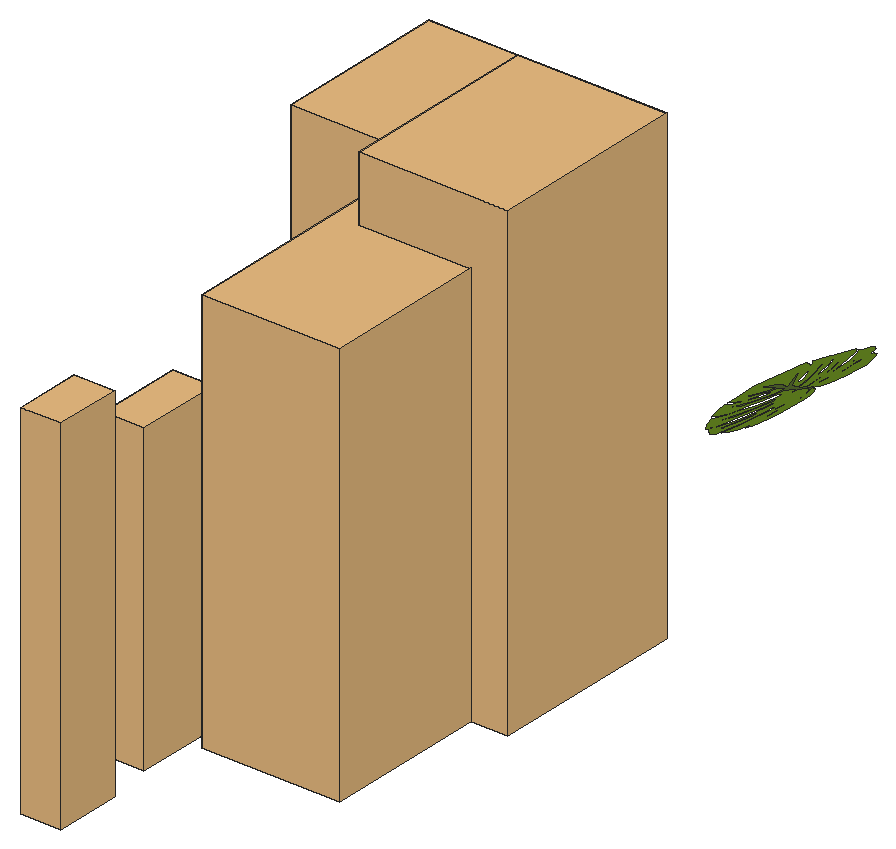
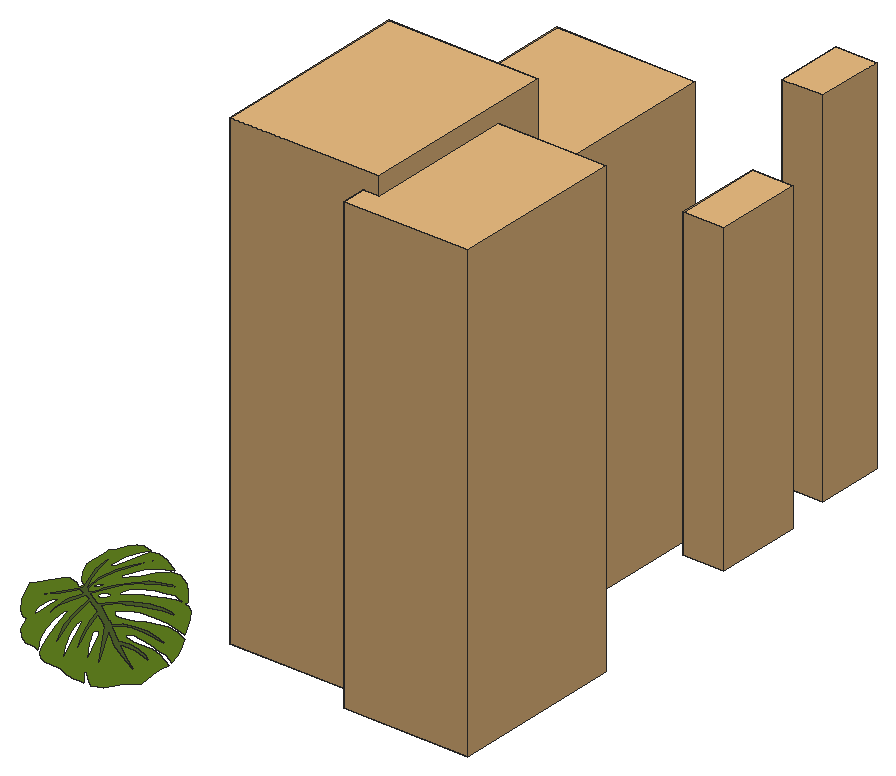
# SketchUp Ruby script. Lengths in inches.
U = 1.inch
M = Sketchup.active_model
def pt(a) = Geom::Point3d.new(a.map { |v| v * U })
def face(e, loops, mat)
  f = e.add_face(loops[0].map { |a| pt(a) })
  loops[1..].each { |l| e.add_face(l.map { |a| pt(a) }).erase! }
  f.material = f.back_material = mat if mat
  f
end
# faces: each face lists its corners as indices into pts; further lists are holes
def faces(e, pts, list, mat = nil) = list.each { |f| face(e, (f[0].is_a?(Array) ? f : [f]).map { |l| l.map { |i| pts[i] } }, mat) }
# xy, xz, yz: faces in a plane at the given z, y or x. An outline is a flat list of corners, or four numbers for a rectangle; further outlines are holes
def ring(l) = l.size == 4 ? [[l[0], l[1]], [l[2], l[1]], [l[2], l[3]], [l[0], l[3]]] : l.each_slice(2).to_a
def flat(e, list, mat, &to3) = list.each { |f| face(e, (f[0].is_a?(Array) ? f : [f]).map { |l| ring(l).map { |u, v| to3.(u, v) } }, mat) }
def xy(e, z, list, mat = nil) = flat(e, list, mat) { |x, y| [x, y, z] }
def xz(e, y, list, mat = nil) = flat(e, list, mat) { |x, z| [x, y, z] }
def yz(e, x, list, mat = nil) = flat(e, list, mat) { |y, z| [x, y, z] }
def lines(e, pts, list) = list.each { |a, b| e.add_line(pt(pts[a]), pt(pts[b])) }
# prism: a flat outline (further loops are holes) pulled along v
def prism(e, loops, v, mat = nil)
  f = face(e, loops, mat); d = Geom::Vector3d.new(v.map { |x| x * U })
  f.pushpull(f.normal.samedirection?(d) ? d.length : -d.length)
end
def box(e, o, s, mat = nil) = prism(e, [[o, [o[0] + s[0], o[1], o[2]], [o[0] + s[0], o[1] + s[1], o[2]], [o[0], o[1] + s[1], o[2]]]], [0, 0, s[2]], mat)
def at(x, y, z, deg = 0) = Geom::Transformation.translation(pt([x, y, z])) * Geom::Transformation.rotation(ORIGIN, Z_AXIS, deg.degrees)
def axes(o, x, y, z) = Geom::Transformation.new([*x, 0, *y, 0, *z, 0, *pt(o).to_a, 1])
def part(name) = M.definitions.add(name)
# library, detail: a bought-in or finely detailed component or shape, given as its bounding box
def library(name, o, s) = part(name).tap { |d| box(d.entities, o, s) }
def detail(e, o, s) = box(e.add_group.entities, o, s)
def put(e, d, t, mat = nil) = e.add_instance(d, t).tap { |i| i.material = mat if mat }
def group(e, t, mat = nil) = e.add_group.tap { |g| g.transformation = t; g.material = mat if mat }.entities
root = M.entities
M.materials.add("[0059_DarkOliveGreen]").color = [85, 107, 47]
M.materials.add("[0061_OliveDrab]").color = [107, 142, 35]
c1 = library("EXOTIC-PEONY",[-0.63,-0.48,-0.08],[13.23,10.24,55.71])
c2 = library("EXOTIC-RED-POKER\#1",[-1.18,-1.18,0],[10.24,10.24,66.04])
c3 = library("EXOTICA-CAT-TAIL",[-18.64,-20.64,0],[26.41,31.25,82.25])
c4 = library("EXOTIC-BAMBOO",[-8.14,-8.14,0],[38.48,34.74,73.65])
c5 = library("EXOTIC-BAMBOO-TOO",[-9.25,-15.15,0],[30.31,37.46,85.46])
p = [[300.68,91.1875,26.91],[300.57,90.58,26.85],[301.02,90.23,27.08],[301.65,89.36,27.4],[302.04,88.16,27.6],[302.1,86.89,27.63],
  [302.04,85.61,27.6],[302.09,84.71,27.62],[301.77,83.65,27.46],[301.54,82.48,27.34],[301.15,81.46,27.15],[300.68,80.95,26.91],
  [300,80.7,26.56],[300.21,81.47,26.67],[300.48,82.51,26.81],[300.7,83.8,26.92],[300.83,85.63,26.99],[300.82,85.94,26.98],
  [300.67,86.03,26.9],[300.54,85.72,26.84],[300.38,84.69,26.76],[300.26,83.26,26.7],[299.99,81.49,26.5625],[299.89,80.92,26.51],
  [299.39,80.3125,26.26],[298.5,80.1,25.81],[297.26,80.46,25.18],[298.28,82.12,25.7],[298.82,83.32,25.97],[299.28,85.14,26.2],
  [299.37,86.05,26.25],[299.28,86.26,26.2],[299.1,86.03,26.11],[298.92,85.41,26.02],[298.47,84.05,25.79],[298.03,82.48,25.57],
  [297.32,81.02,25.21],[296.71,80.39,24.9],[295.62,80.625,24.35],[294.96,81.31,24.02],[294.23,82.125,23.65],[294.08,82.44,23.57],
  [294.29,82.8,23.68],[294.79,82.82,23.93],[295.17,82.96,24.13],[295.84,83.54,24.46],[296.53,84.29,24.8125],[297.58,85.77,25.34],
  [297.97,86.72,25.54],[298.09,87.53,25.6],[298.07,87.98,25.59],[297.86,87.94,25.48],[297.69,87.54,25.4],[297.31,86.81,25.21],
  [296.81,85.875,24.96],[296.04,84.78,24.57],[295.51,84.06,24.3],[294.875,83.22,23.98],[293.66,82.7,23.36],[293.24,82.91,23.15],
  [292.625,83.96,22.84],[291.67,85.875,22.36],[293.25,86.39,23.16],[294.5,87.09,23.79],[295.52,87.9,24.3],[296.32,88.89,24.71],
  [296.67,89.64,24.88],[296.87,90.27,24.99],[296.65,90.59,24.875],[296.3125,90.54,24.7],[295.83,90.05,24.46],[295.25,89.29,24.17],
  [294.59,88.34,23.83],[293.625,87.25,23.35],[293.06,86.76,23.06],[292.27,86.41,22.66],[291.2,86.44,22.125],[290.97,87.03,22.01],
  [290.75,87.49,21.89],[290.5,88.1,21.77],[290.26,88.87,21.64],[290.08,89.94,21.56],[290.51,89.78,21.77],[290.98,89.73,22.01],
  [291.53,89.94,22.29],[292.45,90.18,22.75],[293.51,90.53,23.29],[293.96,90.82,23.51],[294.4,91.29,23.74],[294.49,91.55,23.78],
  [294.39,91.72,23.73],[294.05,91.67,23.5625],[293.64,91.61,23.35],[293.01,91.11,23.04],[292.09,90.47,22.57],[291.26,90.34,22.15],
  [289.97,90.52,21.5],[290.01,91.46,21.52],[290,93.02,21.52],[289.79,94.92,21.41],[290.81,97.07,21.93],[291.35,98.88,22.2],
  [291.74,99.41,22.4],[292.14,99.93,22.6],[292.38,99.9,22.72],[293.87,98.72,23.47],[293.22,99.68,23.14],[292.78,100.3,22.92],
  [293.08,100.48,23.07],[293.6,100.88,23.34],[294.22,101.11,23.65],[294.88,101.1,23.98],[295.17,101.27,24.125],[295.73,101.61,24.41],
  [296.37,101.93,24.73],[296.82,102.01,24.96],[297.3,101.58,25.2],[297.66,100.75,25.38],[298.22,99.01,25.67],[298.68,97.28,25.9],
  [299.08,95.14,26.1],[299.2,94.75,26.16],[299.29,94.77,26.21],[299.33,95.16,26.23],[299.25,96.75,26.1875],[298.89,98.52,26.01],
  [298.37,100.14,25.74],[297.67,101.4,25.39],[297.98,101.44,25.54],[298.78,101.78,25.95],[299.39,101.65,26.26],[300.15,100.89,26.64],
  [300.57,99.39,26.86],[301.02,99.46,27.08],[301.66,99.11,27.41],[302.41,97.9375,27.78],[303.37,95.52,28.27],[303.04,94.67,28.1],
  [302.65,93.35,27.91],[302.22,91.93,27.6875],[301.79,91.16,27.47],[301.16,91.0625,27.16],[296.2,92.67,24.65],[293.7,96.79,23.39],
  [295.625,92.74,24.36],[294.3,93.61,23.6875],[293,94.02,23.03],[291.58,94.19,22.3125],[291.45,94.2,22.25],[292.31,93.91,22.68],
  [292.95,93.63,23.01],[294.16,93.14,23.62],[293.58,92.64,23.32],[292.78,92.13,22.92],[291.44,91.92,22.24],[291.99,91.66,22.52],
  [292.79,91.78,22.93],[293.63,92.16,23.35],[294.41,92.86,23.74],[295.85,92.03,24.47],[295.375,91.02,24.23],[294.6875,90.16,23.88],
  [293.78,89.52,23.43],[292.03,88.72,22.54],[293.02,88.87,23.04],[293.81,89.19,23.4375],[294.74,89.82,23.91],[295.54,90.73,24.32],
  [296.01,91.8,24.55],[298,90.95,25.56],[297.37,89.26,25.24],[295.93,87.08,24.51],[294.66,85.62,23.87],[293.79,84.89,23.43],
  [294.18,84.95,23.63],[294.85,85.38,23.96],[295.77,86.15,24.43],[297.29,88.25,25.2],[297.84,89.57,25.47],[298.4,91.01,25.76],
  [299.53,90.73,26.33],[299.02,88.52,26.07],[298.48,86.625,25.8],[297.7,84.74,25.4],[297.13,83.68,25.12],[295.93,82.11,24.51],
  [296.31,82.17,24.71],[296.93,82.99,25.02],[297.71,83.97,25.41],[298.35,85.35,25.73],[299.17,87.77,26.15],[299.4,88.7,26.27],
  [299.49,89.66,26.31],[299.67,90.47,26.4],[299.83,90.62,26.48],[300.03,90.41,26.58],[300.125,89.72,26.63],[300.2,88.31,26.67],
  [299.97,86.1875,26.55],[299.68,84.41,26.41],[299.08,81.59,26.1],[299.375,82.35,26.25],[299.84,84.03,26.49],[300.21,85.81,26.67],
  [300.45,88.41,26.79],[300.19,90.34,26.67],[300.54,89.43,26.84],[301.01,87.58,27.08],[301.41,85.07,27.28],[301.4375,86.21,27.29],
  [301.28,87.85,27.21],[300.68,89.88,26.91],[300.45,90.92,26.79],[302.14,96.12,27.65],[301.09,93.83,27.12],[300.38,91.45,26.76],
  [299.97,91.39,26.55],[299.95,91.78,26.54],[300.36,93.36,26.75],[300.25,95.54,26.69],[299.82,97.98,26.47],[300.11,94.95,26.625],
  [299.8125,92.92,26.47],[299.59,91.38,26.36],[299.18,91.55,26.15],[298.87,93.96,25.99],[298.34,96.54,25.73],[297.07,99.64,25.09],
  [298.3,95.18,25.71],[298.9,91.71,26.01],[297.8125,91.98,25.46],[297.45,93.43,25.28],[296.59,95.91,24.84],[295.47,98.28,24.28],
  [296.77,94.7,24.93],[297.41,92.22,25.26],[297.33,96.77,25.22],[296.84,97.91,24.97],[296.5625,98.54,24.83],[295.44,100.46,24.27],
  [295.74,99.71,24.42],[296.39,98.13,24.74],[296.95,96.54,25.03],[297.45,95.1,25.28],[297.67,94.49,25.39],[297.79,94.42,25.45],
  [297.84,94.64,25.48],[297.8,95.16,25.45],[295.91,95.31,24.5],[295.75,95.64,24.42],[295.6,95.95,24.34],[294.43,97.8,23.75],
  [295.01,96.29,24.04],[295.63,94.66,24.36],[295.78,94.25,24.4375],[296.05,93.85,24.57],[296.24,93.78,24.67],[296.36,94.04,24.73],
  [296.23,94.67,24.66],[301.05,96.1,27.1],[301.0625,96.64,27.1],[300.93,97.5625,27.04],[300.63,98.09,26.88],[300.58,97.74,26.86],
  [300.5625,96.3,26.85],[300.61,94.57,26.875],[300.74,94.52,26.94],[300.92,94.76,27.03],[301.04,95.55,27.09],[298.79,90.34,25.95],
  [298.45,89.9,25.79],[298.35,89.26,25.73],[298.47,89,25.79],[298.76,89.16,25.94],[298.99,89.64,26.06],[299.04,90.24,26.08],
  [299.87,89.05,26.5],[299.98,89.49,26.56],[299.87,89.8125,26.5],[299.67,89.44,26.4],[299.5,88.77,26.3125],[299.625,88.53,26.38],
  [299.82,88.86,26.48]]
faces(root,p,[[[0,1,2,3,4,5,6,7,8,9,10,11,12,13,14,15,16,17,18,19,20,21,22,23,24,25,26,27,28,29,30,31,32,33,34,35,36,37,38,39,40,41,42,43,44,45,46,47,48,49,50,51,52,53,54,55,56,57,42,58,59,60,61,62,63,64,65,66,67,68,69,70,71,72,73,74,75,76,77,78,79,80,81,82,83,84,85,86,87,88,89,90,91,92,93,94,95,96,97,98,99,100,101,102,103,104,105,106,107,108,109,110,111,112,113,114,115,116,117,118,119,120,121,122,123,124,125,126,127,128,129,130,131,132,133,134,135,136,137,138,139,140,141],[142,143,144,145,146,147,148,149,150,151,152,153,154,155,156,157,158,159,160,161,162,163,164,165,166,167,168,169,170,171,172,173,174,175,176,177,178,179,180,181,182,183,184,185,186,187,188,189,190,191,192,193,194,195,196,197,198,199,200,201,202,203,204,205,206,207,208,209,210,211,212,213,214,215,216,217,218,219,220,221,222,223,224,225,226,227,228,229,230,231,232,233,234,235],[236,237,238,239,240,241,242,243,244,245,246,247],[248,249,250,251,252,253,254,255,256,257,258],[259,260,261,262,263,264,265,266,267,268],[269,270,271,272,273,274,275],[276,277,278,279,280,281,282]]],"[0061_OliveDrab]")
faces(root,p,[[143,142,235,234,233,232,231,230,229,228,227,226,225,224,223,222,221,220,219,218,217,216,215,214,213,212,211,210,209,208,207,206,205,204,203,202,201,200,199,198,197,196,195,194,193,192,191,190,189,188,187,186,185,184,183,182,181,180,179,178,177,176,175,174,173,172,171,170,169,168,167,166,165,164,163,162,161,160,159,158,157,156,155,154,153,152,151,150,149,148,147,146,145,144]],"[0059_DarkOliveGreen]")
put(root,c1,axes([272.98,24.64,9.51],[0,-0.82,0],[0.49713,0,0],[0,0,0.69]))
put(root,c2,axes([278.3,7.43,9.51],[-0.49713,0,0],[0,-0.82,0],[0,0,0.69]))
put(root,c3,axes([279.4,54.45,9.51],[0,-0.82,0],[0.49713,0,0],[0,0,0.69]))
put(root,c4,axes([283.48,46.2,9.51],[0,-0.82,0],[0.49713,0,0],[0,0,0.69]))
put(root,c5,axes([290.26,59.08,9.51],[0,-0.82,0],[0.49713,0,0],[0,0,0.69]))
